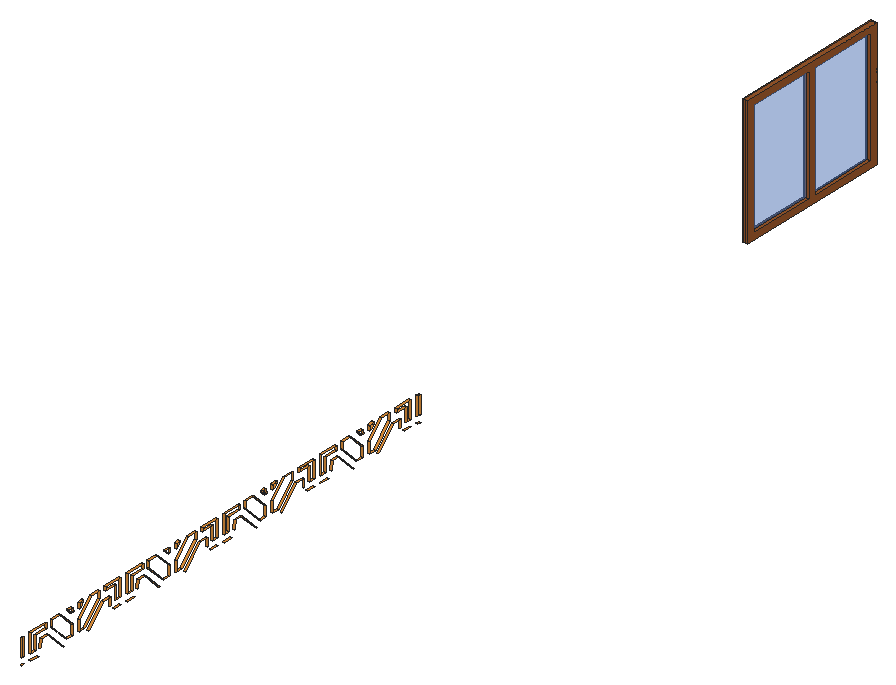
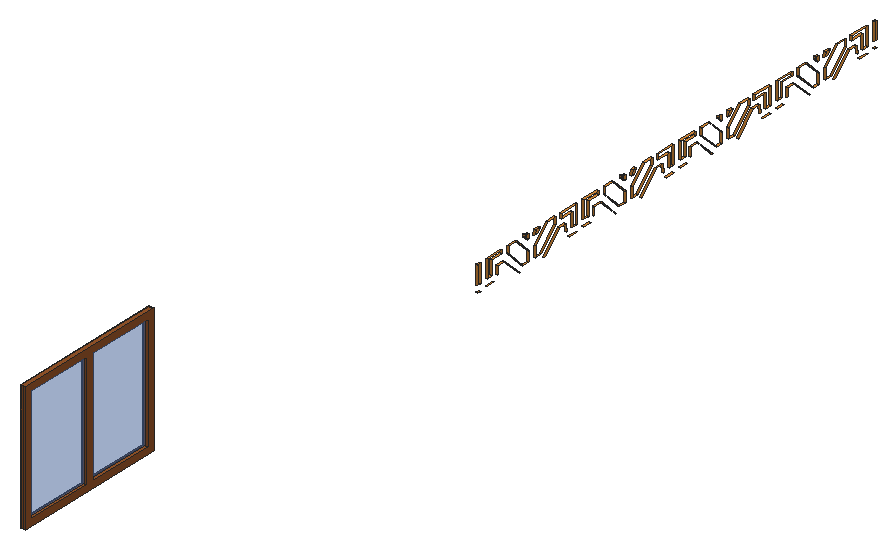
# SketchUp Ruby script. Lengths in inches.
U = 1.inch
M = Sketchup.active_model
def pt(a) = Geom::Point3d.new(a.map { |v| v * U })
def face(e, loops, mat)
  f = e.add_face(loops[0].map { |a| pt(a) })
  loops[1..].each { |l| e.add_face(l.map { |a| pt(a) }).erase! }
  f.material = f.back_material = mat if mat
  f
end
# faces: each face lists its corners as indices into pts; further lists are holes
def faces(e, pts, list, mat = nil) = list.each { |f| face(e, (f[0].is_a?(Array) ? f : [f]).map { |l| l.map { |i| pts[i] } }, mat) }
# xy, xz, yz: faces in a plane at the given z, y or x. An outline is a flat list of corners, or four numbers for a rectangle; further outlines are holes
def ring(l) = l.size == 4 ? [[l[0], l[1]], [l[2], l[1]], [l[2], l[3]], [l[0], l[3]]] : l.each_slice(2).to_a
def flat(e, list, mat, &to3) = list.each { |f| face(e, (f[0].is_a?(Array) ? f : [f]).map { |l| ring(l).map { |u, v| to3.(u, v) } }, mat) }
def xy(e, z, list, mat = nil) = flat(e, list, mat) { |x, y| [x, y, z] }
def xz(e, y, list, mat = nil) = flat(e, list, mat) { |x, z| [x, y, z] }
def yz(e, x, list, mat = nil) = flat(e, list, mat) { |y, z| [x, y, z] }
def lines(e, pts, list) = list.each { |a, b| e.add_line(pt(pts[a]), pt(pts[b])) }
# prism: a flat outline (further loops are holes) pulled along v
def prism(e, loops, v, mat = nil)
  f = face(e, loops, mat); d = Geom::Vector3d.new(v.map { |x| x * U })
  f.pushpull(f.normal.samedirection?(d) ? d.length : -d.length)
end
def box(e, o, s, mat = nil) = prism(e, [[o, [o[0] + s[0], o[1], o[2]], [o[0] + s[0], o[1] + s[1], o[2]], [o[0], o[1] + s[1], o[2]]]], [0, 0, s[2]], mat)
def at(x, y, z, deg = 0) = Geom::Transformation.translation(pt([x, y, z])) * Geom::Transformation.rotation(ORIGIN, Z_AXIS, deg.degrees)
def axes(o, x, y, z) = Geom::Transformation.new([*x, 0, *y, 0, *z, 0, *pt(o).to_a, 1])
def part(name) = M.definitions.add(name)
# library, detail: a bought-in or finely detailed component or shape, given as its bounding box
def library(name, o, s) = part(name).tap { |d| box(d.entities, o, s) }
def detail(e, o, s) = box(e.add_group.entities, o, s)
def put(e, d, t, mat = nil) = e.add_instance(d, t).tap { |i| i.material = mat if mat }
def group(e, t, mat = nil) = e.add_group.tap { |g| g.transformation = t; g.material = mat if mat }.entities
root = M.entities
M.materials.add("1056 AP 9903 Mellow Melon-N").color = [219, 142, 59]
M.materials.add("[Translucent Glass Blue]").color = [100, 149, 237]
M.materials["[Translucent Glass Blue]"].alpha = 0.5
M.materials.add("[Wood Cherry Original]").color = [152, 86, 42]
c1 = part("Group17\#2")
xy(c1.entities,0,[[-27.5,-21.5,-1.25,21.5],[1.25,-21.5,27.5,21.5]])
c2 = part("Group16\#1")
prism(c2.entities,[[[-30,-24,0],[-30,24,0],[30,24,0],[30,-24,0]],[[-27.5,-21.5,0],[-1.25,-21.5,0],[-1.25,21.5,0],[-27.5,21.5,0]],[[27.5,-21.5,0],[27.5,21.5,0],[1.25,21.5,0],[1.25,-21.5,0]]],[0,0,2])
put(c2.entities,c1,at(0,0,1),"[Translucent Glass Blue]")
xy(root,158.23,[[14.35,41.65,15.0625,44.2],[14.35,87,15.0625,89.54],[14.35,132.34,15.0625,134.89],[14.35,177.68,15.0625,180.23]],"1056 AP 9903 Mellow Melon-N")
xy(root,158.35,[[14.35,18.88,15.0625,22.375],[14.35,35.75,15.0625,38.38],[14.35,64.22,15.0625,67.72],[14.35,81.09,15.0625,83.72],[14.35,109.57,15.0625,113.0625],
  [14.35,126.4375,15.0625,129.07],[14.35,154.91,15.0625,158.41],[14.35,171.78,15.0625,174.41],[14.35,200.25,15.0625,201.3125]],"1056 AP 9903 Mellow Melon-N")
xy(root,158.67,[[14.35,14.79,15.0625,15.64],[14.35,58.01,15.0625,60.99],[14.35,103.35,15.0625,106.33],[14.35,148.7,15.0625,151.67],[14.35,194.04,15.0625,197.02]],"1056 AP 9903 Mellow Melon-N")
xy(root,160.93,[[14.35,18.88,15.0625,21.05],[14.35,64.22,15.0625,66.39],[14.35,109.57,15.0625,111.73],[14.35,154.91,15.0625,157.08],[14.35,200.25,15.0625,201.3125]],"1056 AP 9903 Mellow Melon-N")
xy(root,161.27,[[14.35,14.79,15.0625,15.64],[14.35,58.84,15.0625,60.99],[14.35,104.18,15.0625,106.33],[14.35,149.53,15.0625,151.67],[14.35,194.87,15.0625,197.02]],"1056 AP 9903 Mellow Melon-N")
xy(root,163.43,[[14.35,52.85,15.0625,56.26],[14.35,98.2,15.0625,101.6],[14.35,143.54,15.0625,146.95],[14.35,188.88,15.0625,192.29]],"1056 AP 9903 Mellow Melon-N")
xy(root,163.51,[[14.35,24.08,15.0625,27.14],[14.35,69.42,15.0625,72.49],[14.35,114.77,15.0625,117.83],[14.35,160.11,15.0625,163.17]],"1056 AP 9903 Mellow Melon-N")
xy(root,166.04,[[14.35,41.65,15.0625,42.08],[14.35,87,15.0625,87.42],[14.35,132.34,15.0625,132.76],[14.35,177.68,15.0625,178.11]],"1056 AP 9903 Mellow Melon-N")
xy(root,166.08,[[14.35,21.05,15.0625,26.25],[14.35,37.94,15.0625,38.8125],[14.35,66.39,15.0625,71.59],[14.35,83.29,15.0625,84.16],[14.35,111.73,15.0625,116.93],
  [14.35,128.63,15.0625,129.5],[14.35,157.08,15.0625,162.28],[14.35,173.97,15.0625,174.84]],"1056 AP 9903 Mellow Melon-N")
xy(root,166.47,[[14.35,54.11,15.0625,58.84],[14.35,99.46,15.0625,104.18],[14.35,144.8,15.0625,149.53],[14.35,190.14,15.0625,194.87]],"1056 AP 9903 Mellow Melon-N")
xy(root,167.77,[[14.35,14.79,15.0625,15.64],[14.35,47.26,15.0625,51.11],[14.35,54.11,15.0625,60.99],[14.35,92.61,15.0625,96.45],[14.35,99.46,15.0625,106.33],
  [14.35,137.95,15.0625,141.79],[14.35,144.8,15.0625,151.67],[14.35,183.29,15.0625,187.14],[14.35,190.14,15.0625,197.02]],"1056 AP 9903 Mellow Melon-N")
xy(root,167.8,[[14.35,18.88,15.0625,26.25],[14.35,28.85,15.0625,32.77],[14.35,36.65,15.0625,38.38],[14.35,64.22,15.0625,71.59],[14.35,74.19,15.0625,78.11],
  [14.35,81.99,15.0625,83.72],[14.35,109.57,15.0625,116.93],[14.35,119.53,15.0625,123.46],[14.35,127.33,15.0625,129.07],[14.35,154.91,15.0625,162.28],
  [14.35,164.88,15.0625,168.8],[14.35,172.68,15.0625,174.41],[14.35,200.25,15.0625,201.3125]],"1056 AP 9903 Mellow Melon-N")
xz(root,14.79,[[14.35,161.27,15.0625,167.77]],"1056 AP 9903 Mellow Melon-N")
xz(root,15.64,[[14.35,161.27,15.0625,167.77]],"1056 AP 9903 Mellow Melon-N")
xz(root,18.88,[[14.35,160.93,15.0625,167.8]],"1056 AP 9903 Mellow Melon-N")
xz(root,21.05,[[14.35,160.93,15.0625,166.08]],"1056 AP 9903 Mellow Melon-N")
xz(root,26.25,[[14.35,166.08,15.0625,167.8]],"1056 AP 9903 Mellow Melon-N")
xz(root,28.85,[[14.35,165.25,15.0625,167.8]],"1056 AP 9903 Mellow Melon-N")
xz(root,36.65,[[14.35,167.38,15.0625,167.8]],"1056 AP 9903 Mellow Melon-N")
xz(root,38.38,[[14.35,158.35,15.0625,162.19]],"1056 AP 9903 Mellow Melon-N")
xz(root,41.65,[[14.35,158.23,15.0625,162.16],[14.35,166.04,15.0625,167.77]],"1056 AP 9903 Mellow Melon-N")
xz(root,43.37,[[14.35,167.33,15.0625,168.2]],"1056 AP 9903 Mellow Melon-N")
xz(root,51.11,[[14.35,165.14,15.0625,167.77]],"1056 AP 9903 Mellow Melon-N")
xz(root,54.11,[[14.35,166.47,15.0625,167.77]],"1056 AP 9903 Mellow Melon-N")
xz(root,56.26,[[14.35,160.37,15.0625,163.43]],"1056 AP 9903 Mellow Melon-N")
xz(root,58.84,[[14.35,161.27,15.0625,166.47]],"1056 AP 9903 Mellow Melon-N")
xz(root,60.99,[[14.35,161.27,15.0625,167.77]],"1056 AP 9903 Mellow Melon-N")
xz(root,64.22,[[14.35,160.93,15.0625,167.8]],"1056 AP 9903 Mellow Melon-N")
xz(root,66.39,[[14.35,160.93,15.0625,166.08]],"1056 AP 9903 Mellow Melon-N")
xz(root,71.59,[[14.35,166.08,15.0625,167.8]],"1056 AP 9903 Mellow Melon-N")
xz(root,74.19,[[14.35,165.25,15.0625,167.8]],"1056 AP 9903 Mellow Melon-N")
xz(root,81.99,[[14.35,167.38,15.0625,167.8]],"1056 AP 9903 Mellow Melon-N")
xz(root,83.72,[[14.35,158.35,15.0625,162.19]],"1056 AP 9903 Mellow Melon-N")
xz(root,87,[[14.35,158.23,15.0625,162.16],[14.35,166.04,15.0625,167.77]],"1056 AP 9903 Mellow Melon-N")
xz(root,88.72,[[14.35,167.33,15.0625,168.2]],"1056 AP 9903 Mellow Melon-N")
xz(root,96.45,[[14.35,165.14,15.0625,167.77]],"1056 AP 9903 Mellow Melon-N")
xz(root,99.46,[[14.35,166.47,15.0625,167.77]],"1056 AP 9903 Mellow Melon-N")
xz(root,101.6,[[14.35,160.37,15.0625,163.43]],"1056 AP 9903 Mellow Melon-N")
xz(root,104.18,[[14.35,161.27,15.0625,166.47]],"1056 AP 9903 Mellow Melon-N")
xz(root,106.33,[[14.35,161.27,15.0625,167.77]],"1056 AP 9903 Mellow Melon-N")
xz(root,109.57,[[14.35,160.93,15.0625,167.8]],"1056 AP 9903 Mellow Melon-N")
xz(root,111.73,[[14.35,160.93,15.0625,166.08]],"1056 AP 9903 Mellow Melon-N")
xz(root,116.93,[[14.35,166.08,15.0625,167.8]],"1056 AP 9903 Mellow Melon-N")
xz(root,119.53,[[14.35,165.25,15.0625,167.8]],"1056 AP 9903 Mellow Melon-N")
xz(root,127.33,[[14.35,167.38,15.0625,167.8]],"1056 AP 9903 Mellow Melon-N")
xz(root,129.07,[[14.35,158.35,15.0625,162.19]],"1056 AP 9903 Mellow Melon-N")
xz(root,132.34,[[14.35,158.23,15.0625,162.16],[14.35,166.04,15.0625,167.77]],"1056 AP 9903 Mellow Melon-N")
xz(root,134.06,[[14.35,167.33,15.0625,168.2]],"1056 AP 9903 Mellow Melon-N")
xz(root,141.79,[[14.35,165.14,15.0625,167.77]],"1056 AP 9903 Mellow Melon-N")
xz(root,144.8,[[14.35,166.47,15.0625,167.77]],"1056 AP 9903 Mellow Melon-N")
xz(root,146.95,[[14.35,160.37,15.0625,163.43]],"1056 AP 9903 Mellow Melon-N")
xz(root,149.53,[[14.35,161.27,15.0625,166.47]],"1056 AP 9903 Mellow Melon-N")
xz(root,151.67,[[14.35,161.27,15.0625,167.77]],"1056 AP 9903 Mellow Melon-N")
xz(root,154.91,[[14.35,160.93,15.0625,167.8]],"1056 AP 9903 Mellow Melon-N")
xz(root,157.08,[[14.35,160.93,15.0625,166.08]],"1056 AP 9903 Mellow Melon-N")
xz(root,162.28,[[14.35,166.08,15.0625,167.8]],"1056 AP 9903 Mellow Melon-N")
xz(root,164.88,[[14.35,165.25,15.0625,167.8]],"1056 AP 9903 Mellow Melon-N")
xz(root,172.68,[[14.35,167.38,15.0625,167.8]],"1056 AP 9903 Mellow Melon-N")
xz(root,174.41,[[14.35,158.35,15.0625,162.19]],"1056 AP 9903 Mellow Melon-N")
xz(root,177.68,[[14.35,158.23,15.0625,162.16],[14.35,166.04,15.0625,167.77]],"1056 AP 9903 Mellow Melon-N")
xz(root,179.4,[[14.35,167.33,15.0625,168.2]],"1056 AP 9903 Mellow Melon-N")
xz(root,187.14,[[14.35,165.14,15.0625,167.77]],"1056 AP 9903 Mellow Melon-N")
xz(root,190.14,[[14.35,166.47,15.0625,167.77]],"1056 AP 9903 Mellow Melon-N")
xz(root,192.29,[[14.35,160.37,15.0625,163.43]],"1056 AP 9903 Mellow Melon-N")
xz(root,194.87,[[14.35,161.27,15.0625,166.47]],"1056 AP 9903 Mellow Melon-N")
xz(root,197.02,[[14.35,161.27,15.0625,167.77]],"1056 AP 9903 Mellow Melon-N")
xz(root,200.25,[[14.35,160.93,15.0625,167.8]],"1056 AP 9903 Mellow Melon-N")
xz(root,201.3125,[[14.35,160.93,15.0625,167.8]],"1056 AP 9903 Mellow Melon-N")
p = [[15.0625,52.85,163.43],[15.0625,45.95,156.53],[14.35,45.95,156.53],[14.35,52.85,163.43],[15.0625,98.2,163.43],[15.0625,91.29,156.53],
  [14.35,91.29,156.53],[14.35,98.2,163.43],[15.0625,143.54,163.43],[15.0625,136.64,156.53],[14.35,136.64,156.53],[14.35,143.54,163.43],
  [15.0625,188.88,163.43],[15.0625,181.98,156.53],[14.35,181.98,156.53],[14.35,188.88,163.43],[15.0625,34.05,156.6],[15.0625,27.14,163.51],
  [14.35,27.14,163.51],[14.35,34.05,156.6],[15.0625,79.39,156.6],[15.0625,72.49,163.51],[14.35,72.49,163.51],[14.35,79.39,156.6],
  [15.0625,124.73,156.6],[15.0625,117.83,163.51],[14.35,117.83,163.51],[14.35,124.73,156.6],[15.0625,170.08,156.6],[15.0625,163.17,163.51],
  [14.35,163.17,163.51],[14.35,170.08,156.6],[15.0625,44.2,158.23],[15.0625,51.11,165.14],[14.35,51.11,165.14],[14.35,44.2,158.23],
  [15.0625,89.54,158.23],[15.0625,96.45,165.14],[14.35,96.45,165.14],[14.35,89.54,158.23],[15.0625,134.89,158.23],[15.0625,141.79,165.14],
  [14.35,141.79,165.14],[14.35,134.89,158.23],[15.0625,180.23,158.23],[15.0625,187.14,165.14],[14.35,187.14,165.14],[14.35,180.23,158.23],
  [15.0625,28.85,165.25],[15.0625,35.75,158.35],[14.35,35.75,158.35],[14.35,28.85,165.25],[15.0625,74.19,165.25],[15.0625,81.09,158.35],
  [14.35,81.09,158.35],[14.35,74.19,165.25],[15.0625,119.53,165.25],[15.0625,126.4375,158.35],[14.35,126.4375,158.35],[14.35,119.53,165.25],
  [15.0625,164.88,165.25],[15.0625,171.78,158.35],[14.35,171.78,158.35],[14.35,164.88,165.25],[15.0625,24.08,163.51],[15.0625,23.65,160.53],
  [14.35,23.65,160.53],[14.35,24.08,163.51],[15.0625,69.42,163.51],[15.0625,68.99,160.53],[14.35,68.99,160.53],[14.35,69.42,163.51],
  [15.0625,114.77,163.51],[15.0625,114.34,160.53],[14.35,114.34,160.53],[14.35,114.77,163.51],[15.0625,160.11,163.51],[15.0625,159.68,160.53],
  [14.35,159.68,160.53],[14.35,160.11,163.51],[15.0625,38.38,162.19],[15.0625,32.77,167.8],[14.35,32.77,167.8],[14.35,38.38,162.19],
  [15.0625,47.26,167.77],[15.0625,41.65,162.16],[14.35,41.65,162.16],[14.35,47.26,167.77],[15.0625,83.72,162.19],[15.0625,78.11,167.8],
  [14.35,78.11,167.8],[14.35,83.72,162.19],[15.0625,92.61,167.77],[15.0625,87,162.16],[14.35,87,162.16],[14.35,92.61,167.77],
  [15.0625,129.07,162.19],[15.0625,123.46,167.8],[14.35,123.46,167.8],[14.35,129.07,162.19],[15.0625,137.95,167.77],[15.0625,132.34,162.16],
  [14.35,132.34,162.16],[14.35,137.95,167.77],[15.0625,174.41,162.19],[15.0625,168.8,167.8],[14.35,168.8,167.8],[14.35,174.41,162.19],
  [15.0625,183.29,167.77],[15.0625,177.68,162.16],[14.35,177.68,162.16],[14.35,183.29,167.77],[15.0625,42.08,166.04],[15.0625,43.37,167.33],
  [14.35,43.37,167.33],[14.35,42.08,166.04],[15.0625,87.42,166.04],[15.0625,88.72,167.33],[14.35,88.72,167.33],[14.35,87.42,166.04],
  [15.0625,132.76,166.04],[15.0625,134.06,167.33],[14.35,134.06,167.33],[14.35,132.76,166.04],[15.0625,178.11,166.04],[15.0625,179.4,167.33],
  [14.35,179.4,167.33],[14.35,178.11,166.04],[15.0625,36.65,167.38],[15.0625,37.94,166.08],[14.35,37.94,166.08],[14.35,36.65,167.38],
  [15.0625,38.8125,166.08],[15.0625,38.38,167.8],[14.35,38.38,167.8],[14.35,38.8125,166.08],[15.0625,81.99,167.38],[15.0625,83.29,166.08],
  [14.35,83.29,166.08],[14.35,81.99,167.38],[15.0625,84.16,166.08],[15.0625,83.72,167.8],[14.35,83.72,167.8],[14.35,84.16,166.08],
  [15.0625,127.33,167.38],[15.0625,128.63,166.08],[14.35,128.63,166.08],[14.35,127.33,167.38],[15.0625,129.5,166.08],[15.0625,129.07,167.8],
  [14.35,129.07,167.8],[14.35,129.5,166.08],[15.0625,172.68,167.38],[15.0625,173.97,166.08],[14.35,173.97,166.08],[14.35,172.68,167.38],
  [15.0625,174.84,166.08],[15.0625,174.41,167.8],[14.35,174.41,167.8],[14.35,174.84,166.08],[15.0625,43.37,168.2],[15.0625,41.65,167.77],
  [14.35,41.65,167.77],[14.35,43.37,168.2],[15.0625,88.72,168.2],[15.0625,87,167.77],[14.35,87,167.77],[14.35,88.72,168.2],
  [15.0625,134.06,168.2],[15.0625,132.34,167.77],[14.35,132.34,167.77],[14.35,134.06,168.2],[15.0625,179.4,168.2],[15.0625,177.68,167.77],
  [14.35,177.68,167.77],[14.35,179.4,168.2],[26.375,399.5625,210],[26.375,399.5625,162],[26.375,339.5625,162],[26.375,339.5625,210]]
faces(root,p,[[0,1,2,3],[4,5,6,7],[8,9,10,11],[12,13,14,15],[16,17,18,19],[20,21,22,23],[24,25,26,27],[28,29,30,31],
  [32,33,34,35],[36,37,38,39],[40,41,42,43],[44,45,46,47],[48,49,50,51],[52,53,54,55],[56,57,58,59],[60,61,62,63],
  [64,65,66,67],[68,69,70,71],[72,73,74,75],[76,77,78,79],[80,81,82,83],[84,85,86,87],[88,89,90,91],[92,93,94,95],
  [96,97,98,99],[100,101,102,103],[104,105,106,107],[108,109,110,111],[112,113,114,115],[116,117,118,119],[120,121,122,123],[124,125,126,127],
  [128,129,130,131],[132,133,134,135],[136,137,138,139],[140,141,142,143],[144,145,146,147],[148,149,150,151],[152,153,154,155],[156,157,158,159],
  [160,161,162,163],[164,165,166,167],[168,169,170,171],[172,173,174,175]],"1056 AP 9903 Mellow Melon-N")
lines(root,p,[[176,177],[177,178],[178,179]])
put(root,c2,axes([27.375,369.5625,186],[0,-1,0],[0,0,1],[-1,0,0]),"[Wood Cherry Original]")
